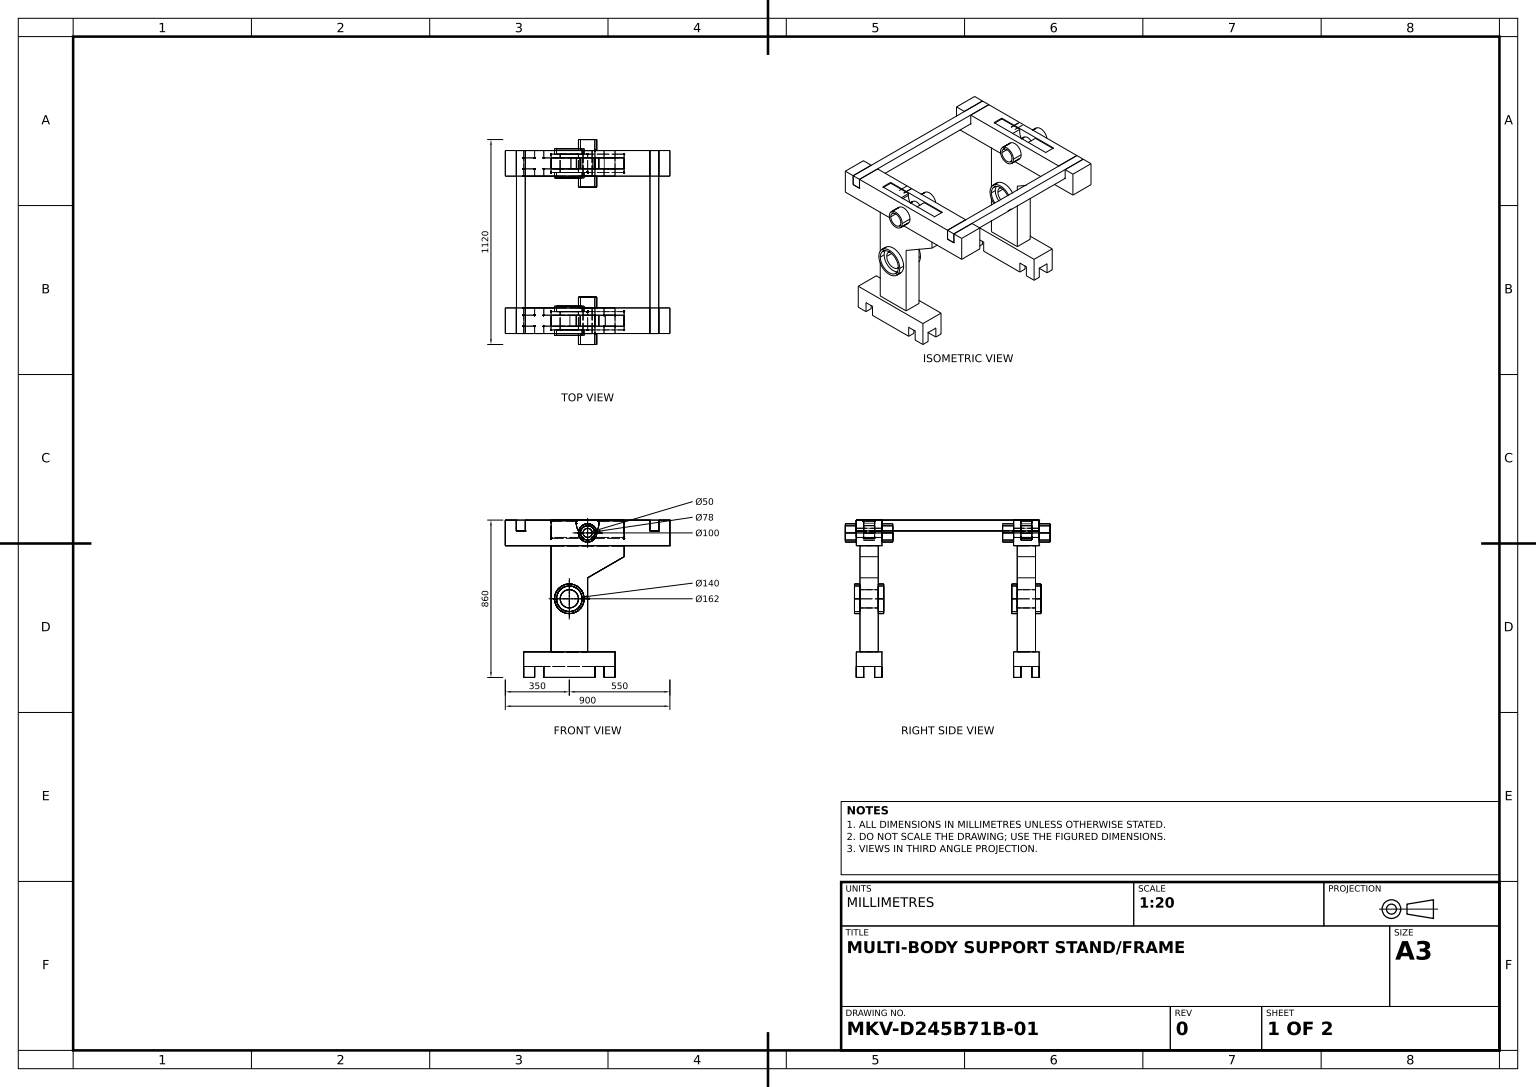
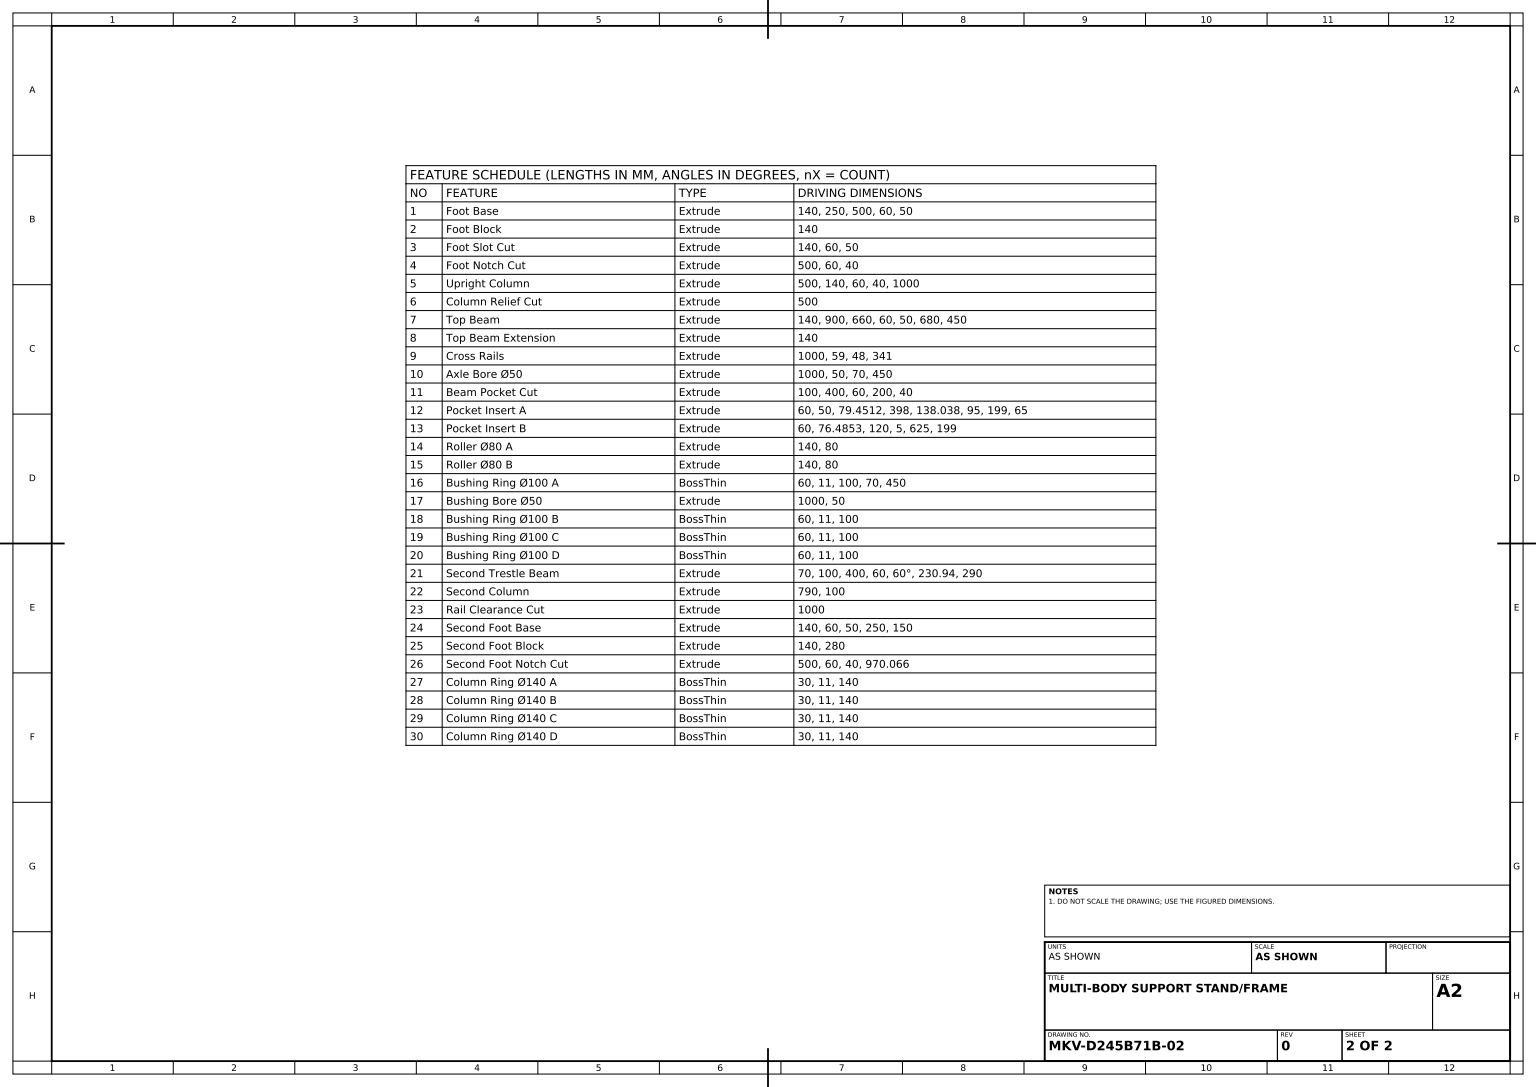
solid
v1 (40,790,820)
v2 (-40,790,820)
e1 v1 v2 CIRCLE(AX(P(0,790,820),D(0,0,1),D(1,0,0)),40)
v3 (40,790,760)
e2 v3 v1 LINE
v4 (-40,790,760)
e3 v3 v4 CIRCLE(AX(P(0,790,760),D(0,0,1),D(1,0,0)),40)
e4 v4 v2 LINE
face CYL(AX(P(0,790,720),D(0,0,1),D(1,0,0)),40) [-e1 -e2 e3 e4]
v5 (90,60,720)
v6 (90,0,720)
e5 v5 v6 LINE
v7 (90,0,760)
e6 v6 v7 LINE
v8 (90,60,760)
e7 v8 v7 LINE
e8 v5 v8 LINE
face PLANE(AX(P(90,60,720),D(-1,0,0),D(0,0,1))) [e5 e6 -e7 -e8]
v9 (340,800,720)
v10 (340,800,860)
e9 v9 v10 LINE
v11 (390,800,860)
e10 v11 v10 LINE
v12 (390,800,720)
e11 v12 v11 LINE
e12 v12 v9 LINE
face PLANE(AX(P(390,800,720),D(0,1,0),D(0,0,1))) [e9 -e10 -e11 e12]
v13 (150,0,820)
v14 (150,60,820)
e13 v13 v14 LINE
v15 (150,60,760)
e14 v14 v15 LINE
v16 (150,0,760)
e15 v15 v16 LINE
v17 (150,0,720)
e16 v17 v16 LINE
v18 (150,140,720)
e17 v17 v18 LINE
v19 (150,140,860)
e18 v18 v19 LINE
v20 (150,0,860)
e19 v20 v19 LINE
e20 v13 v20 LINE
face PLANE(AX(P(150,0,720),D(1,0,0),D(0,0,-1))) [e13 e14 e15 -e16 e17 e18 -e19 -e20]
v21 (40,60,820)
v22 (-240,60,820)
e21 v21 v22 LINE
v23 (40,0,820)
e22 v21 v23 LINE
v24 (-240,0,820)
e23 v23 v24 LINE
e24 v24 v22 LINE
face PLANE(AX(P(150,0,820),D(0,0,1),D(1,0,0))) rev [-e21 e22 e23 e24]
v25 (-39.92763,787.594924,760)
e25 v4 v25 CIRCLE(AX(P(0,790,760),D(0,0,1),D(1,0,0)),40)
v26 (-39.92763,787.594924,820)
e26 v25 v26 LINE
e27 v2 v26 CIRCLE(AX(P(0,790,820),D(0,0,1),D(1,0,0)),40)
face CYL(AX(P(0,790,720),D(0,0,1),D(1,0,0)),40) [e25 e26 -e27 -e4]
v27 (40,60,860)
e28 v21 v27 LINE
v28 (40,0,860)
e29 v28 v27 LINE
e30 v23 v28 LINE
face PLANE(AX(P(40,0,720),D(1,0,0),D(0,0,-1))) [-e22 e28 -e29 -e30]
v29 (-19,430,710)
v30 (-19,430,740)
e31 v29 v30 LINE
v31 (-181,430,710)
e32 v31 v29 CIRCLE(AX(P(-100,430,710),D(0,0,-1),D(-1,0,0)),81)
v32 (-181,430,740)
e33 v31 v32 LINE
e34 v32 v30 CIRCLE(AX(P(-100,430,740),D(0,0,-1),D(-1,0,0)),81)
face CYL(AX(P(-100,430,710),D(0,0,1),D(1,0,0)),81) [-e31 -e32 e33 e34]
v33 (-60.961774,855,820)
v34 (-61.951243,842.5,820)
e35 v33 v34 CIRCLE(AX(P(17.5,842.5,820),D(0,0,1),D(1,0,0)),79.451243)
v35 (-61.951243,842.5,760)
e36 v34 v35 LINE
v36 (-60.961774,855,760)
e37 v36 v35 CIRCLE(AX(P(17.5,842.5,760),D(0,0,1),D(1,0,0)),79.451243)
e38 v33 v36 LINE
face CYL(AX(P(17.5,842.5,820),D(0,0,-1),D(-1,0,0)),79.451243) rev [e35 e36 -e37 -e38]
v37 (-50,430,740)
v38 (-150,430,740)
e39 v37 v38 CIRCLE(AX(P(-100,430,740),D(0,0,1),D(1,0,0)),50)
e40 v38 v37 CIRCLE(AX(P(-100,430,740),D(0,0,1),D(1,0,0)),50)
v39 (-30,430,740)
v40 (-170,430,740)
e41 v39 v40 CIRCLE(AX(P(-100,430,740),D(0,0,1),D(-1,0,0)),70)
e42 v40 v39 CIRCLE(AX(P(-100,430,740),D(0,0,1),D(-1,0,0)),70)
face PLANE(AX(P(0,0,740),D(0,0,-1),D(-1,0,0))) [e39 e40] [-e41 -e42]
v41 (-39,790,660)
v42 (-39,790,720)
e43 v41 v42 LINE
v43 (39,790,660)
e44 v41 v43 CIRCLE(AX(P(0,790,660),D(0,0,-1),D(-1,0,0)),39)
v44 (39,790,720)
e45 v43 v44 LINE
e46 v42 v44 CIRCLE(AX(P(0,790,720),D(0,0,-1),D(-1,0,0)),39)
face CYL(AX(P(0,790,660),D(0,0,1),D(1,0,0)),39) rev [-e43 e44 e45 -e46]
v45 (90,0,820)
v46 (90,0,860)
e47 v45 v46 LINE
v47 (90,60,860)
e48 v47 v46 LINE
v48 (90,60,820)
e49 v48 v47 LINE
e50 v45 v48 LINE
face PLANE(AX(P(90,60,720),D(-1,0,0),D(0,0,1))) [e47 -e48 -e49 -e50]
v49 (199,855,820)
v50 (199,855,760)
e51 v49 v50 LINE
v51 (199,760,820)
e52 v49 v51 LINE
v52 (199,760,760)
e53 v51 v52 LINE
e54 v50 v52 LINE
face PLANE(AX(P(199,0,820),D(1,0,0),D(0,0,-1))) [-e51 e52 e53 -e54]
v53 (-200,760,760)
v54 (-200,760,820)
e55 v53 v54 LINE
v55 (-199,760,820)
e56 v54 v55 LINE
v56 (-199,760,760)
e57 v55 v56 LINE
e58 v53 v56 LINE
face PLANE(AX(P(0,760,0),D(0,1,0),D(0,0,1))) [e55 e56 e57 -e58]
v57 (340,860,720)
e59 v9 v57 LINE
v58 (340,860,860)
e60 v57 v58 LINE
e61 v10 v58 LINE
face PLANE(AX(P(340,800,720),D(1,0,0),D(0,0,-1))) [e59 e60 -e61 -e9]
v59 (39,790,920)
v60 (39,790,860)
e62 v59 v60 LINE
v61 (-39,790,920)
e63 v59 v61 CIRCLE(AX(P(0,790,920),D(0,0,1),D(1,0,0)),39)
v62 (-39,790,860)
e64 v61 v62 LINE
e65 v62 v60 CIRCLE(AX(P(0,790,860),D(0,0,-1),D(1,0,0)),39)
face CYL(AX(P(0,790,920),D(0,0,-1),D(-1,0,0)),39) rev [-e62 e63 e64 e65]
v63 (-30,430,870)
v64 (-170,430,870)
e66 v63 v64 CIRCLE(AX(P(-100,430,870),D(0,0,1),D(1,0,0)),70)
e67 v64 v63 CIRCLE(AX(P(-100,430,870),D(0,0,1),D(1,0,0)),70)
v65 (-19,430,870)
v66 (-181,430,870)
e68 v65 v66 CIRCLE(AX(P(-100,430,870),D(0,0,1),D(1,0,0)),81)
e69 v66 v65 CIRCLE(AX(P(-100,430,870),D(0,0,1),D(1,0,0)),81)
face PLANE(AX(P(-100,430,870),D(0,0,1),D(1,0,0))) [-e66 -e67] [e68 e69]
e70 v44 v42 CIRCLE(AX(P(0,790,720),D(0,0,-1),D(-1,0,0)),39)
v67 (25,790,720)
v68 (-25,790,720)
e71 v67 v68 CIRCLE(AX(P(0,790,720),D(0,0,1),D(1,0,0)),25)
e72 v68 v67 CIRCLE(AX(P(0,790,720),D(0,0,1),D(1,0,0)),25)
face PLANE(AX(P(0,0,720),D(0,0,1),D(1,0,0))) rev [e70 e46] [e71 e72]
v69 (-240,0,860)
e73 v24 v69 LINE
v70 (-240,60,860)
e74 v70 v69 LINE
e75 v22 v70 LINE
face PLANE(AX(P(-240,60,720),D(-1,0,0),D(0,0,1))) [-e24 e73 -e74 -e75]
v71 (-340,800,720)
v72 (-340,800,860)
e76 v71 v72 LINE
v73 (-390,800,720)
e77 v71 v73 LINE
v74 (-390,800,860)
e78 v73 v74 LINE
e79 v72 v74 LINE
face PLANE(AX(P(-390,800,720),D(0,1,0),D(0,0,1))) [-e76 e77 e78 -e79]
v75 (-450,720,860)
v76 (450,720,860)
e80 v75 v76 LINE
v77 (450,860,860)
e81 v76 v77 LINE
v78 (390,860,860)
e82 v77 v78 LINE
e83 v78 v11 LINE
v79 (-340,860,860)
e84 v58 v79 LINE
e85 v79 v72 LINE
v80 (-390,860,860)
e86 v74 v80 LINE
v81 (-450,860,860)
e87 v80 v81 LINE
e88 v81 v75 LINE
v82 (50,790,860)
v83 (-50,790,860)
e89 v82 v83 CIRCLE(AX(P(0,790,860),D(0,0,1),D(1,0,0)),50)
e90 v83 v82 CIRCLE(AX(P(0,790,860),D(0,0,1),D(1,0,0)),50)
face PLANE(AX(P(0,0,860),D(0,0,1),D(1,0,0))) [e80 e81 e82 e83 e10 e61 e84 e85 e79 e86 e87 e88] [-e89 -e90]
v84 (390,860,720)
e91 v84 v78 LINE
e92 v84 v12 LINE
face PLANE(AX(P(390,860,720),D(-1,0,0),D(0,0,1))) [-e83 -e91 e92 e11]
v85 (-340,860,720)
e93 v85 v79 LINE
e94 v85 v71 LINE
face PLANE(AX(P(-340,800,720),D(-1,0,0),D(0,0,1))) [e76 -e85 -e93 e94]
v86 (450,720,720)
e95 v86 v76 LINE
v87 (450,860,720)
e96 v86 v87 LINE
e97 v87 v77 LINE
face PLANE(AX(P(450,720,720),D(1,0,0),D(0,0,-1))) [-e95 e96 e97 -e81]
v88 (-450,860,720)
v89 (-450,720,720)
e98 v88 v89 LINE
e99 v89 v75 LINE
e100 v88 v81 LINE
face PLANE(AX(P(-450,720,720),D(-1,0,0),D(0,0,1))) [e98 e99 -e88 -e100]
v90 (-25,790,860)
e101 v68 v90 LINE
v91 (25,790,860)
e102 v90 v91 CIRCLE(AX(P(0,790,860),D(0,0,1),D(1,0,0)),25)
e103 v67 v91 LINE
face CYL(AX(P(0,790,-140),D(0,0,1),D(1,0,0)),25) rev [-e72 e101 e102 -e103]
v92 (-50,790,660)
v93 (-50,790,720)
e104 v92 v93 LINE
v94 (50,790,660)
e105 v94 v92 CIRCLE(AX(P(0,790,660),D(0,0,-1),D(-1,0,0)),50)
v95 (50,790,720)
e106 v94 v95 LINE
e107 v95 v93 CIRCLE(AX(P(0,790,720),D(0,0,-1),D(1,0,0)),50)
face CYL(AX(P(0,790,660),D(0,0,1),D(1,0,0)),50) [-e104 -e105 e106 e107]
e108 v92 v94 CIRCLE(AX(P(0,790,660),D(0,0,-1),D(-1,0,0)),50)
e109 v93 v95 CIRCLE(AX(P(0,790,720),D(0,0,-1),D(1,0,0)),50)
face CYL(AX(P(0,790,660),D(0,0,1),D(1,0,0)),50) [-e106 -e108 e104 e109]
v96 (-240,0,720)
v97 (40,0,720)
e110 v96 v97 LINE
v98 (-240,60,720)
e111 v98 v96 LINE
v99 (-290,60,720)
e112 v99 v98 LINE
v100 (-290,0,720)
e113 v100 v99 LINE
v101 (-350,0,720)
e114 v101 v100 LINE
v102 (-350,140,720)
e115 v102 v101 LINE
e116 v18 v102 LINE
e117 v6 v17 LINE
v103 (40,60,720)
e118 v103 v5 LINE
e119 v97 v103 LINE
face PLANE(AX(P(0,0,720),D(0,0,-1),D(-1,0,0))) [-e110 -e111 -e112 -e113 -e114 -e115 -e116 -e17 -e117 -e5 -e118 -e119]
v104 (-200,860,820)
v105 (200,860,820)
e120 v104 v105 LINE
v106 (200,760,820)
e121 v106 v105 LINE
e122 v51 v106 LINE
v107 (60.961774,855,820)
e123 v107 v49 LINE
v108 (39.92763,787.594924,820)
e124 v108 v107 CIRCLE(AX(P(-17.5,842.5,820),D(0,0,1),D(1,0,0)),79.451243)
e125 v108 v1 CIRCLE(AX(P(0,790,820),D(0,0,1),D(1,0,0)),40)
e126 v34 v26 CIRCLE(AX(P(17.5,842.5,820),D(0,0,1),D(1,0,0)),79.451243)
v109 (-199,855,820)
e127 v109 v33 LINE
e128 v109 v55 LINE
e129 v54 v104 LINE
face PLANE(AX(P(0,760,820),D(0,0,1),D(1,0,0))) rev [e120 -e121 -e122 -e52 -e123 -e124 e125 e1 e27 -e126 -e35 -e127 e128 -e56 e129]
v110 (39.92763,787.594924,760)
e130 v108 v110 LINE
v111 (60.961774,855,760)
e131 v107 v111 LINE
e132 v110 v111 CIRCLE(AX(P(-17.5,842.5,760),D(0,0,1),D(1,0,0)),79.451243)
face CYL(AX(P(-17.5,842.5,820),D(0,0,-1),D(-1,0,0)),79.451243) rev [-e130 e124 e131 -e132]
v112 (200,860,760)
e133 v112 v105 LINE
v113 (-200,860,760)
e134 v113 v104 LINE
e135 v113 v112 LINE
e136 v57 v85 LINE
face PLANE(AX(P(340,860,720),D(0,1,0),D(0,0,1))) [e133 -e120 -e134 e135] [e93 -e84 -e60 e136]
v114 (-30,430,840)
v115 (-170,430,840)
e137 v114 v115 CIRCLE(AX(P(-100,430,840),D(0,0,1),D(1,0,0)),70)
e138 v63 v114 LINE
e139 v64 v115 LINE
face CYL(AX(P(-100,430,870),D(0,0,-1),D(-1,0,0)),70) rev [-e137 -e138 e66 e139]
v116 (-290,0,760)
v117 (-290,60,760)
e140 v116 v117 LINE
e141 v100 v116 LINE
e142 v99 v117 LINE
face PLANE(AX(P(-290,0,720),D(1,0,0),D(0,0,-1))) [-e140 -e141 e113 e142]
v118 (-240,60,760)
v119 (-240,0,760)
e143 v118 v119 LINE
v120 (40,0,760)
e144 v120 v119 LINE
v121 (40,60,760)
e145 v120 v121 LINE
e146 v121 v118 LINE
face PLANE(AX(P(150,60,760),D(0,0,-1),D(-1,0,0))) rev [e143 -e144 e145 e146]
e147 v115 v114 CIRCLE(AX(P(-100,430,840),D(0,0,1),D(1,0,0)),70)
face CYL(AX(P(-100,430,870),D(0,0,-1),D(-1,0,0)),70) rev [-e139 e67 e138 -e147]
e148 v87 v84 LINE
e149 v89 v86 LINE
v122 (-390,860,720)
e150 v122 v88 LINE
e151 v73 v122 LINE
face PLANE(AX(P(0,0,720),D(0,0,1),D(1,0,0))) rev [-e77 -e94 -e136 -e59 -e12 -e92 -e148 -e96 -e149 -e98 -e150 -e151] [-e107 -e109]
e152 v53 v113 LINE
face PLANE(AX(P(-200,760,0),D(-1,0,0),D(0,0,1))) rev [e134 -e129 -e55 e152]
v123 (-19,430,840)
e153 v65 v123 LINE
v124 (-181,430,840)
e154 v66 v124 LINE
e155 v124 v123 CIRCLE(AX(P(-100,430,840),D(0,0,1),D(-1,0,0)),81)
face CYL(AX(P(-100,430,870),D(0,0,-1),D(-1,0,0)),81) [-e153 -e69 e154 e155]
v125 (-350,140,860)
v126 (-350,0,860)
e156 v125 v126 LINE
e157 v102 v125 LINE
v127 (-350,0,760)
e158 v101 v127 LINE
v128 (-350,60,760)
e159 v128 v127 LINE
v129 (-350,60,820)
e160 v129 v128 LINE
v130 (-350,0,820)
e161 v130 v129 LINE
e162 v130 v126 LINE
face PLANE(AX(P(-350,140,720),D(-1,0,0),D(0,0,1))) [-e156 -e157 e115 e158 -e159 -e160 -e161 e162]
v131 (-170,430,710)
v132 (-30,430,710)
e163 v131 v132 CIRCLE(AX(P(-100,430,710),D(0,0,-1),D(-1,0,0)),70)
e164 v132 v39 LINE
e165 v131 v40 LINE
face CYL(AX(P(-100,430,710),D(0,0,1),D(1,0,0)),70) rev [e163 e164 e41 -e165]
v133 (-50,790,920)
e166 v133 v83 LINE
v134 (50,790,920)
e167 v134 v82 LINE
e168 v133 v134 CIRCLE(AX(P(0,790,920),D(0,0,1),D(1,0,0)),50)
face CYL(AX(P(0,790,920),D(0,0,-1),D(-1,0,0)),50) [e166 e90 -e167 -e168]
e169 v91 v90 CIRCLE(AX(P(0,790,860),D(0,0,1),D(1,0,0)),25)
face CYL(AX(P(0,790,-140),D(0,0,1),D(1,0,0)),25) rev [-e101 -e71 e103 e169]
v135 (-200,720,840)
v136 (-200,720,740)
e170 v135 v136 LINE
v137 (-200,140,740)
e171 v136 v137 LINE
v138 (-200,140,840)
e172 v138 v137 LINE
e173 v135 v138 LINE
face PLANE(AX(P(-200,140,840),D(1,0,0),D(0,0,-1))) rev [e170 e171 -e172 -e173]
v139 (-199,855,760)
e174 v139 v56 LINE
e175 v139 v36 LINE
e176 v35 v25 CIRCLE(AX(P(17.5,842.5,760),D(0,0,1),D(1,0,0)),79.451243)
e177 v110 v3 CIRCLE(AX(P(0,790,760),D(0,0,1),D(1,0,0)),40)
e178 v111 v50 LINE
v140 (200,760,760)
e179 v52 v140 LINE
e180 v140 v112 LINE
face PLANE(AX(P(0,760,760),D(0,0,1),D(1,0,0))) [-e174 e175 e37 e176 -e25 -e3 -e177 e132 e178 e54 e179 e180 -e135 -e152 e58]
face CYL(AX(P(0,790,720),D(0,0,1),D(1,0,0)),40) [e177 e2 -e125 e130]
e181 v103 v121 LINE
e182 v15 v8 LINE
e183 v14 v48 LINE
e184 v27 v47 LINE
v141 (-290,60,860)
e185 v141 v70 LINE
v142 (-290,60,820)
e186 v142 v141 LINE
e187 v142 v129 LINE
e188 v117 v128 LINE
e189 v98 v118 LINE
face PLANE(AX(P(40,60,720),D(0,-1,0),D(0,0,-1))) [-e146 -e181 e118 e8 -e182 -e14 e183 e49 -e184 -e28 e21 e75 -e185 -e186 e187 e160 -e188 -e142 e112 e189]
face PLANE(AX(P(450,860,720),D(0,1,0),D(0,0,1))) [e148 e91 -e82 -e97]
e190 v13 v45 LINE
face PLANE(AX(P(150,0,820),D(0,0,1),D(1,0,0))) rev [e50 -e183 -e13 e190]
e191 v109 v139 LINE
face PLANE(AX(P(0,855,820),D(0,1,0),D(0,0,1))) [-e175 -e191 e127 e38]
e192 v46 v20 LINE
face PLANE(AX(P(90,0,720),D(0,-1,0),D(0,0,-1))) [-e47 -e190 e20 -e192]
e193 v30 v32 CIRCLE(AX(P(-100,430,740),D(0,0,-1),D(-1,0,0)),81)
v143 (200,660,740)
v144 (200,720,740)
e194 v143 v144 LINE
v145 (0,544.529946,740)
e195 v145 v143 LINE
v146 (0,140,740)
e196 v146 v145 LINE
e197 v137 v146 LINE
e198 v144 v136 LINE
face PLANE(AX(P(0,0,740),D(0,0,-1),D(-1,0,0))) [-e193 -e34] [-e194 -e195 -e196 -e197 -e171 -e198]
v147 (200,660,840)
e199 v147 v143 LINE
v148 (0,544.529946,840)
e200 v148 v147 LINE
e201 v148 v145 LINE
face PLANE(AX(P(200,660,840),D(-0.5,0.866025404,0),D(-0.866025404,-0.5,0))) rev [-e199 -e200 e201 e195]
v149 (0,140,840)
e202 v149 v148 LINE
e203 v149 v146 LINE
face PLANE(AX(P(0,544.529946,840),D(-1,0,0),D(0,-1,0))) rev [-e201 -e202 e203 e196]
e204 v69 v28 LINE
face PLANE(AX(P(-240,0,720),D(0,-1,0),D(0,0,-1))) [-e23 e30 -e204 -e73]
e205 v19 v125 LINE
v150 (-290,0,860)
e206 v126 v150 LINE
e207 v150 v141 LINE
face PLANE(AX(P(0,0,860),D(0,0,-1),D(-1,0,0))) rev [e185 e74 e204 e29 e184 e48 e192 e19 e205 e156 e206 e207]
face CYL(AX(P(17.5,842.5,820),D(0,0,-1),D(-1,0,0)),79.451243) rev [-e36 e126 -e26 -e176]
e208 v123 v124 CIRCLE(AX(P(-100,430,840),D(0,0,1),D(-1,0,0)),81)
face CYL(AX(P(-100,430,870),D(0,0,-1),D(-1,0,0)),81) [-e68 e153 e208 -e154]
v151 (-290,0,820)
e209 v142 v151 LINE
e210 v151 v130 LINE
face PLANE(AX(P(150,0,820),D(0,0,1),D(1,0,0))) rev [e161 -e187 e209 e210]
e211 v151 v150 LINE
face PLANE(AX(P(-290,0,720),D(1,0,0),D(0,0,-1))) [e186 -e207 -e211 -e209]
face PLANE(AX(P(0,855,820),D(0,1,0),D(0,0,1))) [e123 e51 -e178 -e131]
e212 v138 v149 LINE
face PLANE(AX(P(-350,140,720),D(0,1,0),D(0,0,1))) [e116 e157 -e205 -e18] [-e212 e172 e197 -e203]
e213 v132 v131 CIRCLE(AX(P(-100,430,710),D(0,0,-1),D(-1,0,0)),70)
face CYL(AX(P(-100,430,710),D(0,0,1),D(1,0,0)),70) rev [-e164 e213 e165 e42]
e214 v122 v80 LINE
face PLANE(AX(P(-450,860,720),D(0,1,0),D(0,0,1))) [e150 e100 -e87 -e214]
v152 (-150,430,840)
e215 v152 v38 LINE
v153 (-50,430,840)
e216 v152 v153 CIRCLE(AX(P(-100,430,840),D(0,0,1),D(1,0,0)),50)
e217 v153 v37 LINE
face CYL(AX(P(-100,430,840),D(0,0,-1),D(-1,0,0)),50) rev [-e215 e216 e217 -e40]
e218 v96 v119 LINE
face PLANE(AX(P(-240,60,720),D(-1,0,0),D(0,0,1))) [e111 e218 -e143 -e189]
e219 v60 v62 CIRCLE(AX(P(0,790,860),D(0,0,-1),D(1,0,0)),39)
face PLANE(AX(P(0,0,860),D(0,0,1),D(1,0,0))) [-e219 -e65] [-e102 -e169]
e220 v116 v127 LINE
face PLANE(AX(P(150,60,760),D(0,0,-1),D(-1,0,0))) rev [e188 e159 -e220 e140]
e221 v97 v120 LINE
face PLANE(AX(P(-240,0,720),D(0,-1,0),D(0,0,-1))) [e110 e221 e144 -e218]
v154 (200,720,840)
e222 v154 v135 LINE
e223 v154 v144 LINE
face PLANE(AX(P(450,720,720),D(0,-1,0),D(0,0,-1))) [-e222 e223 e198 -e170] [-e80 -e99 e149 e95]
face PLANE(AX(P(40,0,720),D(1,0,0),D(0,0,-1))) [-e145 -e221 e119 e181]
e224 v16 v7 LINE
face PLANE(AX(P(90,0,720),D(0,-1,0),D(0,0,-1))) [e16 e224 -e6 e117]
e225 v153 v152 CIRCLE(AX(P(-100,430,840),D(0,0,1),D(1,0,0)),50)
face PLANE(AX(P(0,0,840),D(0,0,-1),D(-1,0,0))) rev [-e225 -e216] [e147 e137]
face PLANE(AX(P(-390,860,720),D(1,0,0),D(0,0,-1))) [-e78 e151 e214 -e86]
e226 v43 v41 CIRCLE(AX(P(0,790,660),D(0,0,-1),D(-1,0,0)),39)
face PLANE(AX(P(0,790,660),D(0,0,-1),D(-1,0,0))) [-e44 -e226] [e105 e108]
e227 v29 v31 CIRCLE(AX(P(-100,430,710),D(0,0,-1),D(-1,0,0)),81)
face CYL(AX(P(-100,430,710),D(0,0,1),D(1,0,0)),81) [-e227 e31 e193 -e33]
face CYL(AX(P(0,790,660),D(0,0,1),D(1,0,0)),39) rev [-e45 e226 e43 -e70]
e228 v61 v59 CIRCLE(AX(P(0,790,920),D(0,0,1),D(1,0,0)),39)
face CYL(AX(P(0,790,920),D(0,0,-1),D(-1,0,0)),39) rev [-e64 e228 e62 e219]
e229 v140 v106 LINE
face PLANE(AX(P(200,760,0),D(-1,0,0),D(0,0,1))) [-e133 -e180 e229 e121]
face PLANE(AX(P(150,60,760),D(0,0,-1),D(-1,0,0))) rev [-e224 -e15 e182 e7]
face PLANE(AX(P(0,760,0),D(0,1,0),D(0,0,1))) [e122 -e229 -e179 -e53]
face PLANE(AX(P(-350,0,720),D(0,-1,0),D(0,0,-1))) [-e162 -e210 e211 -e206]
face PLANE(AX(P(-350,0,720),D(0,-1,0),D(0,0,-1))) [-e158 e114 e141 e220]
face PLANE(AX(P(-199,0,820),D(1,0,0),D(0,0,-1))) rev [-e57 -e128 e191 e174]
e230 v134 v133 CIRCLE(AX(P(0,790,920),D(0,0,1),D(1,0,0)),50)
face CYL(AX(P(0,790,920),D(0,0,-1),D(-1,0,0)),50) [e89 -e166 -e230 e167]
face CYL(AX(P(-100,430,840),D(0,0,-1),D(-1,0,0)),50) rev [e215 -e39 -e217 e225]
face PLANE(AX(P(0,790,920),D(0,0,1),D(1,0,0))) [e230 e168] [-e228 -e63]
e231 v147 v154 LINE
face PLANE(AX(P(200,720,840),D(-1,0,0),D(0,0,1))) rev [e194 -e223 -e231 e199]
face PLANE(AX(P(0,0,840),D(0,0,-1),D(-1,0,0))) rev [-e155 -e208] [e212 e202 e200 e231 e222 e173]
face PLANE(AX(P(-100,430,710),D(0,0,-1),D(-1,0,0))) [-e163 -e213] [e227 e32]
solid
v155 (0,544.529946,-20)
v156 (0,544.529946,-120)
e232 v155 v156 LINE
v157 (0,140,-20)
e233 v157 v155 LINE
v158 (0,140,-120)
e234 v157 v158 LINE
e235 v158 v156 LINE
face PLANE(AX(P(0,0,-20),D(-1,0,0),D(0,0,1))) rev [-e232 -e233 e234 e235]
v159 (50,790,60)
v160 (50,790,0)
e236 v159 v160 LINE
v161 (-50,790,60)
e237 v161 v159 CIRCLE(AX(P(0,790,60),D(0,0,1),D(1,0,0)),50)
v162 (-50,790,0)
e238 v161 v162 LINE
e239 v162 v160 CIRCLE(AX(P(0,790,0),D(0,0,1),D(-1,0,0)),50)
face CYL(AX(P(0,790,60),D(0,0,-1),D(-1,0,0)),50) [-e236 -e237 e238 e239]
e240 v160 v162 CIRCLE(AX(P(0,790,0),D(0,0,1),D(-1,0,0)),50)
e241 v159 v161 CIRCLE(AX(P(0,790,60),D(0,0,1),D(1,0,0)),50)
face CYL(AX(P(0,790,60),D(0,0,-1),D(-1,0,0)),50) [e240 -e238 -e241 e236]
v163 (-170,430,-120)
v164 (-30,430,-120)
e242 v163 v164 CIRCLE(AX(P(-100,430,-120),D(0,0,-1),D(-1,0,0)),70)
v165 (-170,430,-150)
e243 v165 v163 LINE
v166 (-30,430,-150)
e244 v165 v166 CIRCLE(AX(P(-100,430,-150),D(0,0,-1),D(-1,0,0)),70)
e245 v166 v164 LINE
face CYL(AX(P(-100,430,-150),D(0,0,1),D(1,0,0)),70) rev [-e242 -e243 e244 e245]
v167 (-181,430,-150)
v168 (-181,430,-120)
e246 v167 v168 LINE
v169 (-19,430,-120)
e247 v168 v169 CIRCLE(AX(P(-100,430,-120),D(0,0,-1),D(1,0,0)),81)
v170 (-19,430,-150)
e248 v170 v169 LINE
e249 v167 v170 CIRCLE(AX(P(-100,430,-150),D(0,0,-1),D(-1,0,0)),81)
face CYL(AX(P(-100,430,-150),D(0,0,1),D(1,0,0)),81) [e246 e247 -e248 -e249]
v171 (-240,60,-100)
v172 (-240,60,-140)
e250 v171 v172 LINE
v173 (-240,0,-140)
e251 v173 v172 LINE
v174 (-240,0,-100)
e252 v174 v173 LINE
e253 v174 v171 LINE
face PLANE(AX(P(-240,60,0),D(-1,0,0),D(0,0,1))) [e250 -e251 -e252 e253]
v175 (150,0,0)
v176 (150,0,-40)
e254 v175 v176 LINE
v177 (90,0,0)
e255 v175 v177 LINE
v178 (90,0,-40)
e256 v177 v178 LINE
e257 v176 v178 LINE
face PLANE(AX(P(90,0,0),D(0,-1,0),D(0,0,-1))) [-e254 e255 e256 -e257]
v179 (-50,430,-20)
v180 (-50,430,-120)
e258 v179 v180 LINE
v181 (-150,430,-20)
e259 v179 v181 CIRCLE(AX(P(-100,430,-20),D(0,0,1),D(1,0,0)),50)
v182 (-150,430,-120)
e260 v181 v182 LINE
e261 v180 v182 CIRCLE(AX(P(-100,430,-120),D(0,0,1),D(1,0,0)),50)
face CYL(AX(P(-100,430,-20),D(0,0,-1),D(-1,0,0)),50) rev [-e258 e259 e260 -e261]
v183 (-19,430,-20)
v184 (-181,430,-20)
e262 v183 v184 CIRCLE(AX(P(-100,430,-20),D(0,0,1),D(1,0,0)),81)
e263 v184 v183 CIRCLE(AX(P(-100,430,-20),D(0,0,1),D(1,0,0)),81)
v185 (200,660,-20)
e264 v185 v155 LINE
v186 (200,720,-20)
e265 v186 v185 LINE
v187 (-200,720,-20)
e266 v186 v187 LINE
v188 (-200,140,-20)
e267 v187 v188 LINE
e268 v188 v157 LINE
face PLANE(AX(P(0,0,-20),D(0,0,1),D(1,0,0))) [-e262 -e263] [e233 -e264 -e265 e266 e267 e268]
v189 (-290,0,0)
v190 (-350,0,0)
e269 v189 v190 LINE
v191 (-350,0,-40)
e270 v190 v191 LINE
v192 (-290,0,-40)
e271 v192 v191 LINE
e272 v189 v192 LINE
face PLANE(AX(P(-350,0,0),D(0,-1,0),D(0,0,-1))) [e269 e270 -e271 -e272]
v193 (39,790,60)
v194 (39,790,0)
e273 v193 v194 LINE
v195 (-39,790,0)
e274 v195 v194 CIRCLE(AX(P(0,790,0),D(0,0,1),D(1,0,0)),39)
v196 (-39,790,60)
e275 v196 v195 LINE
e276 v196 v193 CIRCLE(AX(P(0,790,60),D(0,0,1),D(1,0,0)),39)
face CYL(AX(P(0,790,60),D(0,0,-1),D(-1,0,0)),39) rev [e273 -e274 -e275 e276]
v197 (200,760,-40)
v198 (200,760,-100)
e277 v197 v198 LINE
v199 (200,860,-40)
e278 v197 v199 LINE
v200 (200,860,-100)
e279 v199 v200 LINE
e280 v198 v200 LINE
face PLANE(AX(P(200,760,0),D(1,0,0),D(0,0,-1))) rev [-e277 e278 e279 -e280]
v201 (-200,140,-120)
e281 v188 v201 LINE
e282 v201 v158 LINE
v202 (150,140,0)
v203 (150,140,-140)
e283 v202 v203 LINE
v204 (-350,140,-140)
e284 v204 v203 LINE
v205 (-350,140,0)
e285 v205 v204 LINE
e286 v205 v202 LINE
face PLANE(AX(P(150,140,0),D(0,1,0),D(0,0,1))) [e281 e282 -e234 -e268] [e283 -e284 -e285 e286]
v206 (-60,855,-100)
v207 (-60,855,-40)
e287 v206 v207 LINE
v208 (-199,855,-100)
e288 v206 v208 LINE
v209 (-199,855,-40)
e289 v208 v209 LINE
e290 v207 v209 LINE
face PLANE(AX(P(0,855,-100),D(0,1,0),D(0,0,1))) [-e287 e288 e289 -e290]
v210 (450,860,0)
v211 (450,720,0)
e291 v210 v211 LINE
v212 (450,720,-140)
e292 v211 v212 LINE
v213 (450,860,-140)
e293 v213 v212 LINE
e294 v210 v213 LINE
face PLANE(AX(P(450,860,0),D(1,0,0),D(0,0,-1))) [e291 e292 -e293 -e294]
v214 (-39,790,-200)
v215 (39,790,-200)
e295 v214 v215 CIRCLE(AX(P(0,790,-200),D(0,0,-1),D(-1,0,0)),39)
v216 (39,790,-140)
e296 v215 v216 LINE
v217 (-39,790,-140)
e297 v216 v217 CIRCLE(AX(P(0,790,-140),D(0,0,1),D(-1,0,0)),39)
e298 v214 v217 LINE
face CYL(AX(P(0,790,-200),D(0,0,1),D(1,0,0)),39) rev [e295 e296 e297 -e298]
v218 (-390,800,0)
v219 (-390,800,-140)
e299 v218 v219 LINE
v220 (-340,800,0)
e300 v218 v220 LINE
v221 (-340,800,-140)
e301 v220 v221 LINE
e302 v219 v221 LINE
face PLANE(AX(P(-390,800,0),D(0,1,0),D(0,0,1))) [-e299 e300 e301 -e302]
v222 (-290,60,0)
e303 v222 v189 LINE
v223 (-290,60,-40)
e304 v192 v223 LINE
e305 v222 v223 LINE
face PLANE(AX(P(-290,0,0),D(1,0,0),D(0,0,-1))) [e303 e272 e304 -e305]
v224 (-200,760,-100)
v225 (-200,860,-100)
e306 v224 v225 LINE
v226 (-200,860,-40)
e307 v226 v225 LINE
v227 (-200,760,-40)
e308 v227 v226 LINE
e309 v227 v224 LINE
face PLANE(AX(P(-200,760,0),D(1,0,0),D(0,0,-1))) [e306 -e307 -e308 e309]
v228 (-340,860,0)
v229 (-340,860,-140)
e310 v228 v229 LINE
v230 (340,860,0)
e311 v228 v230 LINE
v231 (340,860,-140)
e312 v230 v231 LINE
e313 v229 v231 LINE
e314 v226 v199 LINE
e315 v225 v200 LINE
face PLANE(AX(P(-340,860,0),D(0,1,0),D(0,0,1))) [-e310 e311 e312 -e313] [-e279 -e314 e307 e315]
v232 (199,855,-100)
v233 (199,765,-100)
e316 v232 v233 LINE
v234 (199,855,-40)
e317 v232 v234 LINE
v235 (199,765,-40)
e318 v234 v235 LINE
e319 v233 v235 LINE
face PLANE(AX(P(199,0,-100),D(-1,0,0),D(0,0,1))) rev [-e316 e317 e318 -e319]
v236 (200,660,-120)
e320 v236 v156 LINE
e321 v185 v236 LINE
face PLANE(AX(P(-235.788383,408.39746,-20),D(0.5,-0.866025404,0),D(0.866025404,0.5,0))) [-e320 -e321 e264 e232]
e322 v194 v195 CIRCLE(AX(P(0,790,0),D(0,0,1),D(1,0,0)),39)
e323 v193 v196 CIRCLE(AX(P(0,790,60),D(0,0,1),D(1,0,0)),39)
face CYL(AX(P(0,790,60),D(0,0,-1),D(-1,0,0)),39) rev [-e322 -e273 e323 e275]
v237 (90,60,0)
v238 (90,60,-40)
e324 v237 v238 LINE
e325 v238 v178 LINE
e326 v177 v237 LINE
face PLANE(AX(P(90,60,0),D(-1,0,0),D(0,0,1))) [e324 e325 -e256 e326]
v239 (-390,860,0)
v240 (-390,860,-140)
e327 v239 v240 LINE
v241 (-450,860,-140)
e328 v241 v240 LINE
v242 (-450,860,0)
e329 v242 v241 LINE
e330 v242 v239 LINE
face PLANE(AX(P(-450,860,0),D(0,1,0),D(0,0,1))) [e327 -e328 -e329 e330]
v243 (40,0,-100)
v244 (40,0,-140)
e331 v243 v244 LINE
e332 v243 v174 LINE
e333 v244 v173 LINE
face PLANE(AX(P(-240,0,0),D(0,-1,0),D(0,0,-1))) [-e331 e332 e252 -e333]
v245 (200,720,-120)
e334 v245 v236 LINE
e335 v186 v245 LINE
face PLANE(AX(P(200,0,-20),D(1,0,0),D(0,0,-1))) [e265 e321 -e334 -e335]
v246 (40,0,-40)
v247 (-240,0,-40)
e336 v246 v247 LINE
v248 (40,0,0)
e337 v248 v246 LINE
v249 (-240,0,0)
e338 v248 v249 LINE
e339 v249 v247 LINE
face PLANE(AX(P(-240,0,0),D(0,-1,0),D(0,0,-1))) [-e336 -e337 e338 e339]
v250 (-19,430,10)
v251 (-181,430,10)
e340 v250 v251 CIRCLE(AX(P(-100,430,10),D(0,0,1),D(1,0,0)),81)
e341 v251 v250 CIRCLE(AX(P(-100,430,10),D(0,0,1),D(1,0,0)),81)
v252 (-170,430,10)
v253 (-30,430,10)
e342 v252 v253 CIRCLE(AX(P(-100,430,10),D(0,0,1),D(1,0,0)),70)
e343 v253 v252 CIRCLE(AX(P(-100,430,10),D(0,0,1),D(1,0,0)),70)
face PLANE(AX(P(-100,430,10),D(0,0,1),D(1,0,0))) [e340 e341] [-e342 -e343]
v254 (150,0,-100)
v255 (150,0,-140)
e344 v254 v255 LINE
v256 (90,0,-100)
e345 v254 v256 LINE
v257 (90,0,-140)
e346 v256 v257 LINE
e347 v255 v257 LINE
face PLANE(AX(P(90,0,0),D(0,-1,0),D(0,0,-1))) [-e344 e345 e346 -e347]
face PLANE(AX(P(0,790,60),D(0,0,1),D(1,0,0))) [-e323 -e276] [e241 e237]
e348 v181 v179 CIRCLE(AX(P(-100,430,-20),D(0,0,1),D(1,0,0)),50)
e349 v182 v180 CIRCLE(AX(P(-100,430,-120),D(0,0,1),D(1,0,0)),50)
face CYL(AX(P(-100,430,-20),D(0,0,-1),D(-1,0,0)),50) rev [e348 e258 -e349 -e260]
v258 (340,800,-140)
e350 v231 v258 LINE
v259 (340,800,0)
e351 v230 v259 LINE
e352 v259 v258 LINE
face PLANE(AX(P(340,860,0),D(1,0,0),D(0,0,-1))) [-e350 -e312 e351 e352]
e353 v190 v205 LINE
v260 (-240,60,0)
e354 v260 v222 LINE
e355 v249 v260 LINE
v261 (40,60,0)
e356 v261 v248 LINE
e357 v237 v261 LINE
e358 v202 v175 LINE
face PLANE(AX(P(0,0,0),D(0,0,1),D(1,0,0))) [-e353 -e269 -e303 -e354 -e355 -e338 -e356 -e357 -e326 -e255 -e358 -e286]
e359 v166 v165 CIRCLE(AX(P(-100,430,-150),D(0,0,-1),D(-1,0,0)),70)
e360 v170 v167 CIRCLE(AX(P(-100,430,-150),D(0,0,-1),D(-1,0,0)),81)
face PLANE(AX(P(-100,430,-150),D(0,0,-1),D(-1,0,0))) [-e244 -e359] [e249 e360]
v262 (-200,720,-120)
e361 v245 v262 LINE
e362 v187 v262 LINE
v263 (-450,720,0)
e363 v211 v263 LINE
v264 (-450,720,-140)
e364 v263 v264 LINE
e365 v212 v264 LINE
face PLANE(AX(P(450,720,0),D(0,-1,0),D(0,0,-1))) [e361 -e362 -e266 e335] [-e292 e363 e364 -e365]
e366 v164 v163 CIRCLE(AX(P(-100,430,-120),D(0,0,-1),D(-1,0,0)),70)
face PLANE(AX(P(0,0,-120),D(0,0,1),D(1,0,0))) rev [e261 e349] [e242 e366]
v265 (-199,765,-100)
v266 (-199,765,-40)
e367 v265 v266 LINE
e368 v266 v209 LINE
e369 v265 v208 LINE
face PLANE(AX(P(-199,0,-100),D(1,0,0),D(0,0,-1))) rev [e367 e368 -e289 -e369]
v267 (-170,430,-20)
e370 v252 v267 LINE
v268 (-30,430,-20)
e371 v267 v268 CIRCLE(AX(P(-100,430,-20),D(0,0,-1),D(1,0,0)),70)
e372 v253 v268 LINE
face CYL(AX(P(-100,430,10),D(0,0,-1),D(-1,0,0)),70) rev [e370 e371 -e372 e343]
e373 v262 v201 LINE
face PLANE(AX(P(-200,0,-20),D(1,0,0),D(0,0,-1))) rev [-e267 e362 e373 -e281]
v269 (-290,0,-100)
v270 (-350,0,-100)
e374 v269 v270 LINE
v271 (-290,60,-100)
e375 v271 v269 LINE
v272 (-350,60,-100)
e376 v271 v272 LINE
e377 v270 v272 LINE
face PLANE(AX(P(150,0,-100),D(0,0,1),D(1,0,0))) [-e374 -e375 e376 -e377]
e378 v239 v218 LINE
e379 v263 v242 LINE
v273 (390,860,0)
e380 v273 v210 LINE
v274 (390,800,0)
e381 v274 v273 LINE
e382 v259 v274 LINE
e383 v220 v228 LINE
face PLANE(AX(P(0,0,0),D(0,0,-1),D(-1,0,0))) rev [-e378 -e330 -e379 -e363 -e291 -e380 -e381 -e382 -e351 -e311 -e383 -e300] [-e239 -e240]
v275 (-25,790,0)
v276 (25,790,0)
e384 v275 v276 CIRCLE(AX(P(0,790,0),D(0,0,-1),D(-1,0,0)),25)
e385 v276 v275 CIRCLE(AX(P(0,790,0),D(0,0,-1),D(-1,0,0)),25)
face PLANE(AX(P(0,0,0),D(0,0,-1),D(-1,0,0))) rev [e384 e385] [e322 e274]
v277 (-240,60,-40)
e386 v260 v277 LINE
e387 v277 v247 LINE
face PLANE(AX(P(-240,60,0),D(-1,0,0),D(0,0,1))) [-e339 e355 e386 e387]
v278 (26.457513,760,-40)
v279 (31.22499,765,-40)
e388 v278 v279 CIRCLE(AX(P(0,790,-40),D(0,0,1),D(1,0,0)),40)
v280 (26.457513,760,-100)
e389 v278 v280 LINE
v281 (31.22499,765,-100)
e390 v280 v281 CIRCLE(AX(P(0,790,-100),D(0,0,1),D(1,0,0)),40)
e391 v281 v279 LINE
face CYL(AX(P(0,790,0),D(0,0,-1),D(-1,0,0)),40) [-e388 e389 e390 e391]
e392 v169 v168 CIRCLE(AX(P(-100,430,-120),D(0,0,-1),D(1,0,0)),81)
face PLANE(AX(P(0,0,-120),D(0,0,1),D(1,0,0))) rev [-e392 -e247] [e320 -e235 -e282 -e373 -e361 e334]
v282 (40,60,-100)
e393 v282 v243 LINE
e394 v282 v171 LINE
face PLANE(AX(P(150,0,-100),D(0,0,1),D(1,0,0))) [-e253 -e332 -e393 e394]
e395 v268 v267 CIRCLE(AX(P(-100,430,-20),D(0,0,-1),D(1,0,0)),70)
face PLANE(AX(P(0,0,-20),D(0,0,1),D(1,0,0))) [-e395 -e371] [-e348 -e259]
v283 (40,60,-140)
e396 v282 v283 LINE
e397 v283 v244 LINE
face PLANE(AX(P(40,0,0),D(1,0,0),D(0,0,-1))) [-e396 e393 e331 -e397]
v284 (-31.22499,765,-40)
e398 v284 v266 LINE
v285 (-31.22499,765,-100)
e399 v285 v265 LINE
e400 v284 v285 LINE
face PLANE(AX(P(0,765,-100),D(0,1,0),D(0,0,1))) rev [e398 -e367 -e399 -e400]
v286 (60,855,-40)
e401 v234 v286 LINE
v287 (61.485293,840,-40)
e402 v286 v287 CIRCLE(AX(P(-15,840,-40),D(0,0,-1),D(-1,0,0)),76.485293)
v288 (39.864413,786.709324,-40)
e403 v287 v288 CIRCLE(AX(P(-15,840,-40),D(0,0,-1),D(-1,0,0)),76.485293)
v289 (40,790,-40)
e404 v288 v289 CIRCLE(AX(P(0,790,-40),D(0,0,1),D(1,0,0)),40)
v290 (-40,790,-40)
e405 v289 v290 CIRCLE(AX(P(0,790,-40),D(0,0,1),D(1,0,0)),40)
v291 (-39.864413,786.709324,-40)
e406 v290 v291 CIRCLE(AX(P(0,790,-40),D(0,0,1),D(1,0,0)),40)
e407 v207 v291 CIRCLE(AX(P(15,840,-40),D(0,0,1),D(-1,0,0)),76.485293)
v292 (-26.457513,760,-40)
e408 v284 v292 CIRCLE(AX(P(0,790,-40),D(0,0,1),D(1,0,0)),40)
e409 v227 v292 LINE
e410 v278 v197 LINE
e411 v235 v279 LINE
face PLANE(AX(P(0,760,-40),D(0,0,1),D(1,0,0))) rev [e401 e402 e403 e404 e405 e406 -e407 e290 -e368 -e398 e408 -e409 e308 e314 -e278 -e410 e388 -e411 -e318]
v293 (-26.457513,760,-100)
e412 v285 v293 CIRCLE(AX(P(0,790,-100),D(0,0,1),D(1,0,0)),40)
e413 v293 v292 LINE
face CYL(AX(P(0,790,0),D(0,0,-1),D(-1,0,0)),40) [-e408 e400 e412 e413]
e414 v251 v184 LINE
e415 v250 v183 LINE
face CYL(AX(P(-100,430,10),D(0,0,-1),D(-1,0,0)),81) [e262 -e414 -e340 e415]
v294 (60,855,-100)
e416 v232 v294 LINE
e417 v294 v286 LINE
face PLANE(AX(P(0,855,-100),D(0,1,0),D(0,0,1))) [e416 e417 -e401 -e317]
v295 (40,60,-40)
e418 v246 v295 LINE
e419 v261 v295 LINE
face PLANE(AX(P(40,0,0),D(1,0,0),D(0,0,-1))) [e418 -e419 e356 e337]
v296 (390,860,-140)
e420 v296 v213 LINE
e421 v273 v296 LINE
face PLANE(AX(P(390,860,0),D(0,1,0),D(0,0,1))) [e380 e294 -e420 -e421]
v297 (150,60,-100)
e422 v254 v297 LINE
v298 (90,60,-100)
e423 v297 v298 LINE
e424 v256 v298 LINE
face PLANE(AX(P(150,0,-100),D(0,0,1),D(1,0,0))) [-e345 e422 e423 -e424]
v299 (25,790,-140)
v300 (-25,790,-140)
e425 v299 v300 CIRCLE(AX(P(0,790,-140),D(0,0,1),D(1,0,0)),25)
e426 v300 v299 CIRCLE(AX(P(0,790,-140),D(0,0,1),D(1,0,0)),25)
e427 v217 v216 CIRCLE(AX(P(0,790,-140),D(0,0,1),D(-1,0,0)),39)
face PLANE(AX(P(0,0,-140),D(0,0,-1),D(-1,0,0))) [e425 e426] [-e297 -e427]
v301 (39.864413,786.709324,-100)
v302 (40,790,-100)
e428 v301 v302 CIRCLE(AX(P(0,790,-100),D(0,0,1),D(1,0,0)),40)
e429 v289 v302 LINE
e430 v301 v288 LINE
face CYL(AX(P(0,790,0),D(0,0,-1),D(-1,0,0)),40) [e428 -e429 -e404 -e430]
face CYL(AX(P(-100,430,-150),D(0,0,1),D(1,0,0)),70) rev [-e366 -e245 e359 e243]
e431 v215 v214 CIRCLE(AX(P(0,790,-200),D(0,0,-1),D(-1,0,0)),39)
v303 (50,790,-200)
v304 (-50,790,-200)
e432 v303 v304 CIRCLE(AX(P(0,790,-200),D(0,0,-1),D(-1,0,0)),50)
e433 v304 v303 CIRCLE(AX(P(0,790,-200),D(0,0,-1),D(-1,0,0)),50)
face PLANE(AX(P(0,790,-200),D(0,0,-1),D(-1,0,0))) [-e431 -e295] [e432 e433]
v305 (61.485293,840,-100)
e434 v294 v305 CIRCLE(AX(P(-15,840,-100),D(0,0,-1),D(-1,0,0)),76.485293)
e435 v305 v287 LINE
face CYL(AX(P(-15,840,-100),D(0,0,1),D(1,0,0)),76.485293) rev [e434 e435 -e402 -e417]
v306 (150,60,-40)
e436 v297 v306 LINE
e437 v203 v255 LINE
e438 v306 v176 LINE
face PLANE(AX(P(150,0,0),D(1,0,0),D(0,0,-1))) [-e436 -e422 e344 -e437 -e283 e358 e254 -e438]
e439 v224 v293 LINE
face PLANE(AX(P(0,760,0),D(0,1,0),D(0,0,1))) [-e309 e409 -e413 -e439]
v307 (-350,60,-40)
e440 v307 v191 LINE
e441 v223 v307 LINE
face PLANE(AX(P(150,0,-40),D(0,0,-1),D(-1,0,0))) [e271 -e440 -e441 -e304]
v308 (-290,60,-140)
e442 v271 v308 LINE
v309 (-290,0,-140)
e443 v269 v309 LINE
e444 v308 v309 LINE
face PLANE(AX(P(-290,0,0),D(1,0,0),D(0,0,-1))) [-e442 e375 e443 -e444]
e445 v280 v198 LINE
face PLANE(AX(P(0,760,0),D(0,1,0),D(0,0,1))) [e277 -e445 -e389 e410]
e446 v233 v281 LINE
v310 (-39.864413,786.709324,-100)
e447 v206 v310 CIRCLE(AX(P(15,840,-100),D(0,0,1),D(-1,0,0)),76.485293)
v311 (-40,790,-100)
e448 v311 v310 CIRCLE(AX(P(0,790,-100),D(0,0,1),D(1,0,0)),40)
e449 v302 v311 CIRCLE(AX(P(0,790,-100),D(0,0,1),D(1,0,0)),40)
e450 v305 v301 CIRCLE(AX(P(-15,840,-100),D(0,0,-1),D(-1,0,0)),76.485293)
face PLANE(AX(P(0,760,-100),D(0,0,1),D(1,0,0))) [-e434 -e416 e316 e446 -e390 e445 e280 -e315 -e306 e439 -e412 e399 e369 -e288 e447 -e448 -e449 -e428 -e450]
e451 v310 v291 LINE
face CYL(AX(P(15,840,-100),D(0,0,1),D(1,0,0)),76.485293) rev [-e447 e287 e407 -e451]
e452 v306 v238 LINE
face PLANE(AX(P(150,0,-40),D(0,0,-1),D(-1,0,0))) [e257 -e325 -e452 e438]
e453 v295 v277 LINE
e454 v272 v307 LINE
e455 v172 v308 LINE
v312 (90,60,-140)
e456 v312 v283 LINE
e457 v298 v312 LINE
face PLANE(AX(P(-290,60,0),D(0,-1,0),D(0,0,-1))) [e357 e419 e453 -e386 e354 e305 e441 -e454 -e376 e442 -e455 -e250 -e394 e396 -e456 -e457 -e423 e436 e452 -e324]
v313 (-50,790,-140)
e458 v304 v313 LINE
v314 (50,790,-140)
e459 v313 v314 CIRCLE(AX(P(0,790,-140),D(0,0,-1),D(-1,0,0)),50)
e460 v303 v314 LINE
face CYL(AX(P(0,790,-200),D(0,0,1),D(1,0,0)),50) [-e433 e458 e459 -e460]
face PLANE(AX(P(0,765,-100),D(0,1,0),D(0,0,1))) rev [-e446 e319 e411 -e391]
v315 (390,800,-140)
e461 v274 v315 LINE
e462 v258 v315 LINE
face PLANE(AX(P(340,800,0),D(0,1,0),D(0,0,1))) [-e352 e382 e461 -e462]
e463 v221 v229 LINE
face PLANE(AX(P(-340,800,0),D(-1,0,0),D(0,0,1))) [e383 e310 -e463 -e301]
face PLANE(AX(P(150,0,-40),D(0,0,-1),D(-1,0,0))) [-e453 -e418 e336 -e387]
e464 v299 v276 LINE
e465 v300 v275 LINE
face CYL(AX(P(0,790,-140),D(0,0,1),D(1,0,0)),25) rev [-e464 -e426 e465 -e385]
e466 v240 v219 LINE
face PLANE(AX(P(-390,860,0),D(1,0,0),D(0,0,-1))) [e299 -e466 -e327 e378]
e467 v257 v312 LINE
v316 (-350,0,-140)
e468 v309 v316 LINE
e469 v316 v204 LINE
face PLANE(AX(P(0,0,-140),D(0,0,1),D(1,0,0))) rev [e437 e347 e467 e456 e397 e333 e251 e455 e444 e468 e469 e284]
face PLANE(AX(P(90,60,0),D(-1,0,0),D(0,0,1))) [e424 e457 -e467 -e346]
face CYL(AX(P(-100,430,-150),D(0,0,1),D(1,0,0)),81) [-e246 -e360 e248 e392]
face CYL(AX(P(0,790,-140),D(0,0,1),D(1,0,0)),25) rev [-e384 -e465 -e425 e464]
face CYL(AX(P(0,790,-200),D(0,0,1),D(1,0,0)),39) rev [e427 -e296 e431 e298]
e470 v290 v311 LINE
face CYL(AX(P(0,790,0),D(0,0,-1),D(-1,0,0)),40) [e470 e448 e451 -e406]
e471 v314 v313 CIRCLE(AX(P(0,790,-140),D(0,0,-1),D(-1,0,0)),50)
e472 v315 v296 LINE
e473 v264 v241 LINE
face PLANE(AX(P(0,0,-140),D(0,0,-1),D(-1,0,0))) [-e459 -e471] [e313 e350 e462 e472 e420 e293 e365 e473 e328 e466 e302 e463]
face PLANE(AX(P(390,800,0),D(-1,0,0),D(0,0,1))) [-e461 e381 e421 -e472]
face CYL(AX(P(-15,840,-100),D(0,0,1),D(1,0,0)),76.485293) rev [-e403 -e435 e450 e430]
face CYL(AX(P(0,790,-200),D(0,0,1),D(1,0,0)),50) [e460 e471 -e458 -e432]
e474 v270 v316 LINE
face PLANE(AX(P(-350,140,0),D(-1,0,0),D(0,0,1))) [-e270 e353 e285 -e469 -e474 e377 e454 e440]
face CYL(AX(P(-100,430,10),D(0,0,-1),D(-1,0,0)),70) rev [e395 -e370 e342 e372]
face CYL(AX(P(-100,430,10),D(0,0,-1),D(-1,0,0)),81) [e263 -e415 -e341 e414]
face PLANE(AX(P(-450,720,0),D(-1,0,0),D(0,0,1))) [e379 e329 -e473 -e364]
face PLANE(AX(P(-350,0,0),D(0,-1,0),D(0,0,-1))) [-e468 -e443 e374 e474]
face CYL(AX(P(0,790,0),D(0,0,-1),D(-1,0,0)),40) [e449 -e470 -e405 e429]
solid
v317 (-389,860,-140)
v318 (-341,860,-140)
e475 v317 v318 LINE
v319 (-341,801,-140)
e476 v318 v319 LINE
v320 (-389,801,-140)
e477 v319 v320 LINE
e478 v320 v317 LINE
face PLANE(AX(P(0,0,-140),D(0,0,1),D(1,0,0))) rev [e475 e476 e477 e478]
v321 (-341,801,860)
e479 v319 v321 LINE
v322 (-389,801,860)
e480 v321 v322 LINE
e481 v320 v322 LINE
face PLANE(AX(P(0,801,-140),D(0,1,0),D(0,0,1))) rev [e479 e480 -e481 -e477]
v323 (-341,860,860)
e482 v318 v323 LINE
e483 v323 v321 LINE
face PLANE(AX(P(-341,0,-140),D(-1,0,0),D(0,0,1))) rev [-e476 e482 e483 -e479]
v324 (-389,860,860)
e484 v324 v323 LINE
e485 v322 v324 LINE
face PLANE(AX(P(0,0,860),D(0,0,1),D(1,0,0))) [-e480 -e483 -e484 -e485]
e486 v317 v324 LINE
face PLANE(AX(P(-389,0,-140),D(1,0,0),D(0,0,-1))) rev [-e486 -e478 e481 e485]
face PLANE(AX(P(0,860,-140),D(0,-1,0),D(0,0,-1))) rev [e486 e484 -e482 -e475]
solid
v325 (341,801,860)
v326 (389,801,860)
e487 v325 v326 LINE
v327 (341,801,-140)
e488 v327 v325 LINE
v328 (389,801,-140)
e489 v327 v328 LINE
e490 v328 v326 LINE
face PLANE(AX(P(0,801,-140),D(0,-1,0),D(0,0,-1))) [-e487 -e488 e489 e490]
v329 (389,860,-140)
v330 (389,860,860)
e491 v329 v330 LINE
e492 v326 v330 LINE
e493 v328 v329 LINE
face PLANE(AX(P(389,0,-140),D(1,0,0),D(0,0,-1))) [e491 -e492 -e490 e493]
v331 (341,860,-140)
e494 v329 v331 LINE
v332 (341,860,860)
e495 v331 v332 LINE
e496 v330 v332 LINE
face PLANE(AX(P(0,860,-140),D(0,1,0),D(0,0,1))) [-e491 e494 e495 -e496]
e497 v331 v327 LINE
e498 v332 v325 LINE
face PLANE(AX(P(341,0,-140),D(-1,0,0),D(0,0,1))) [e497 e488 -e498 -e495]
face PLANE(AX(P(0,0,-140),D(0,0,1),D(1,0,0))) rev [-e489 -e497 -e494 -e493]
face PLANE(AX(P(0,0,860),D(0,0,1),D(1,0,0))) [e492 e496 e498 e487]
